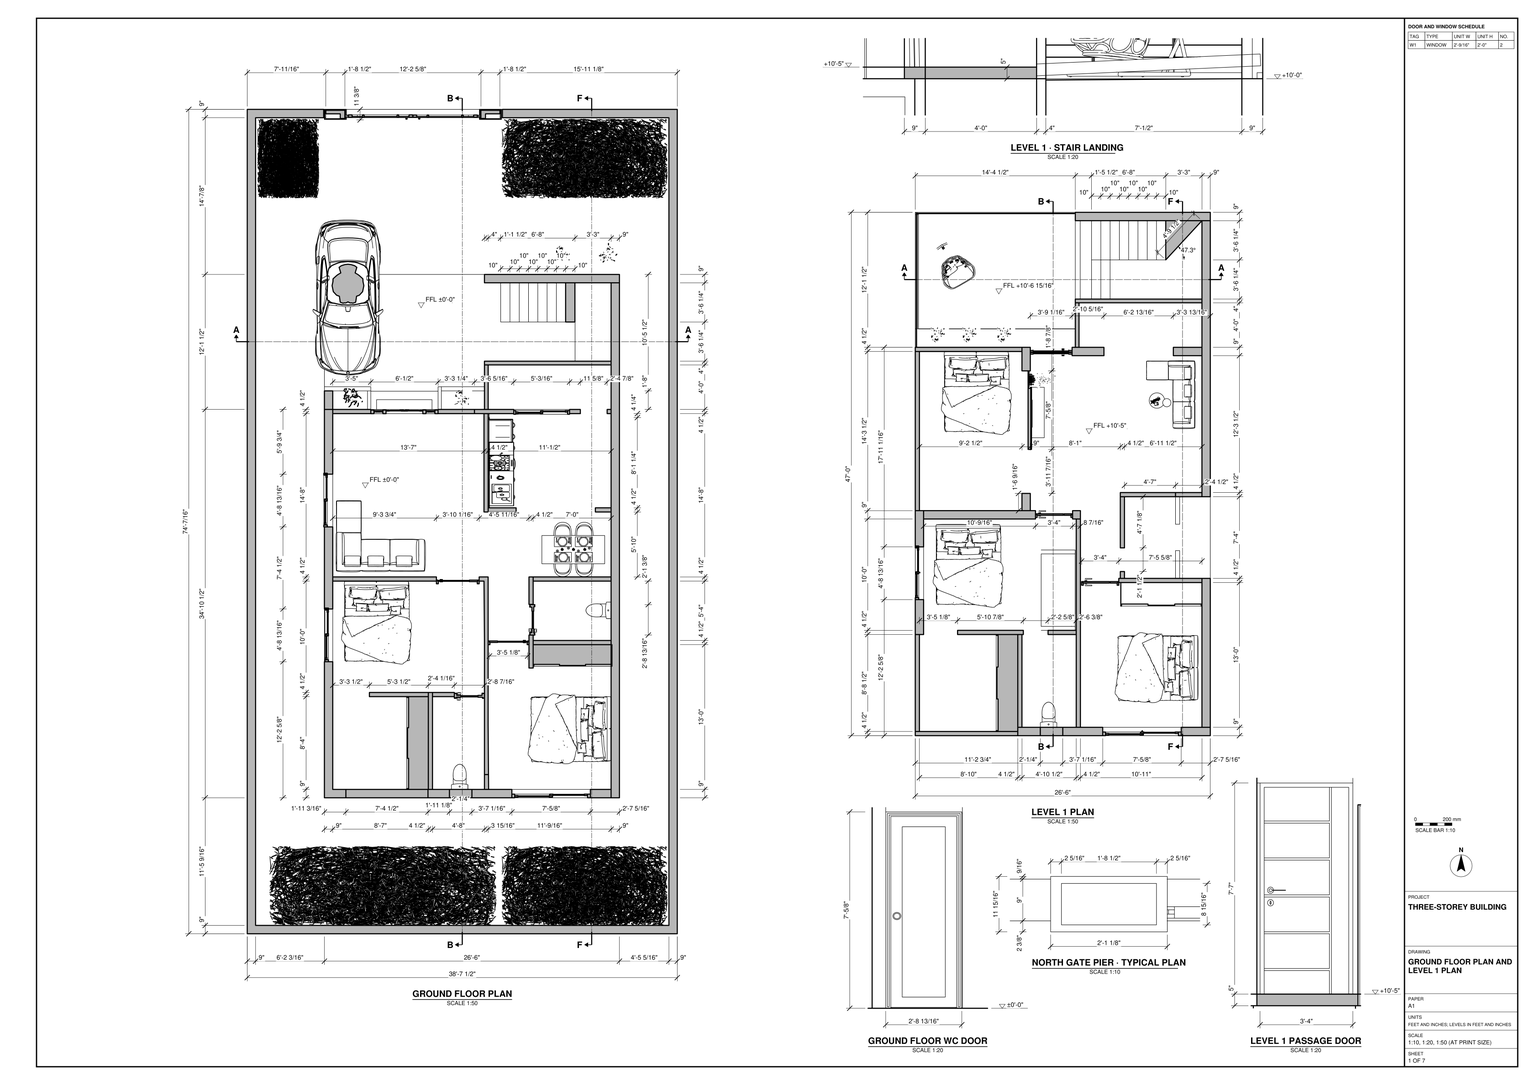
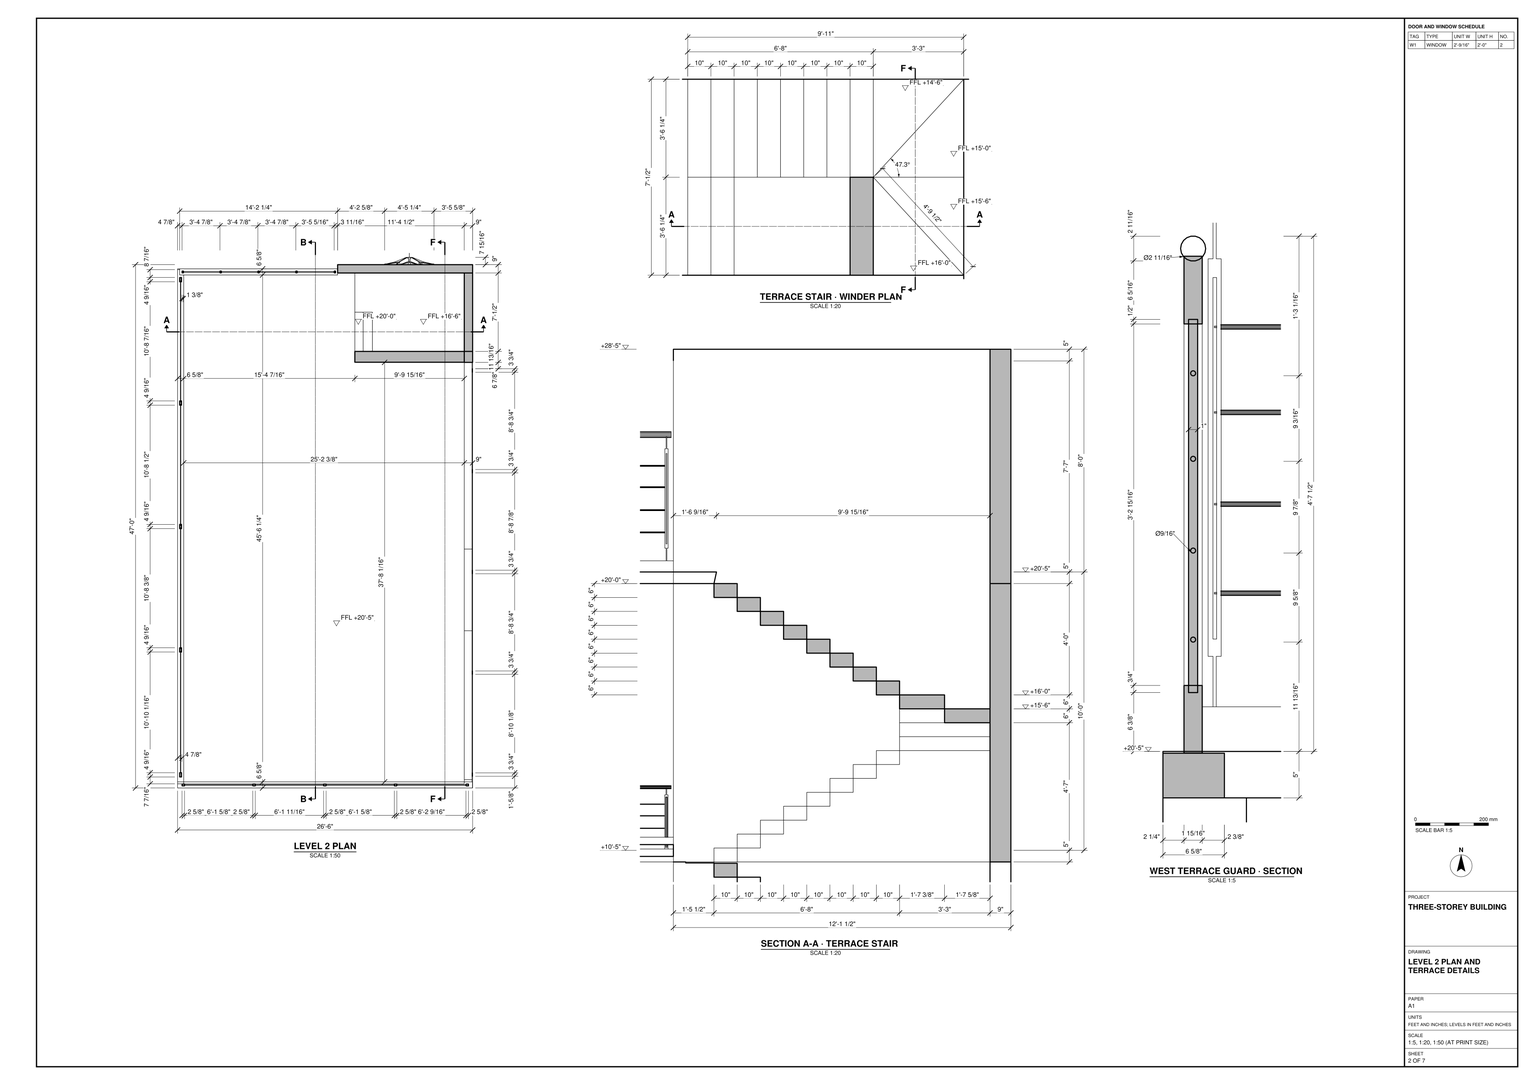
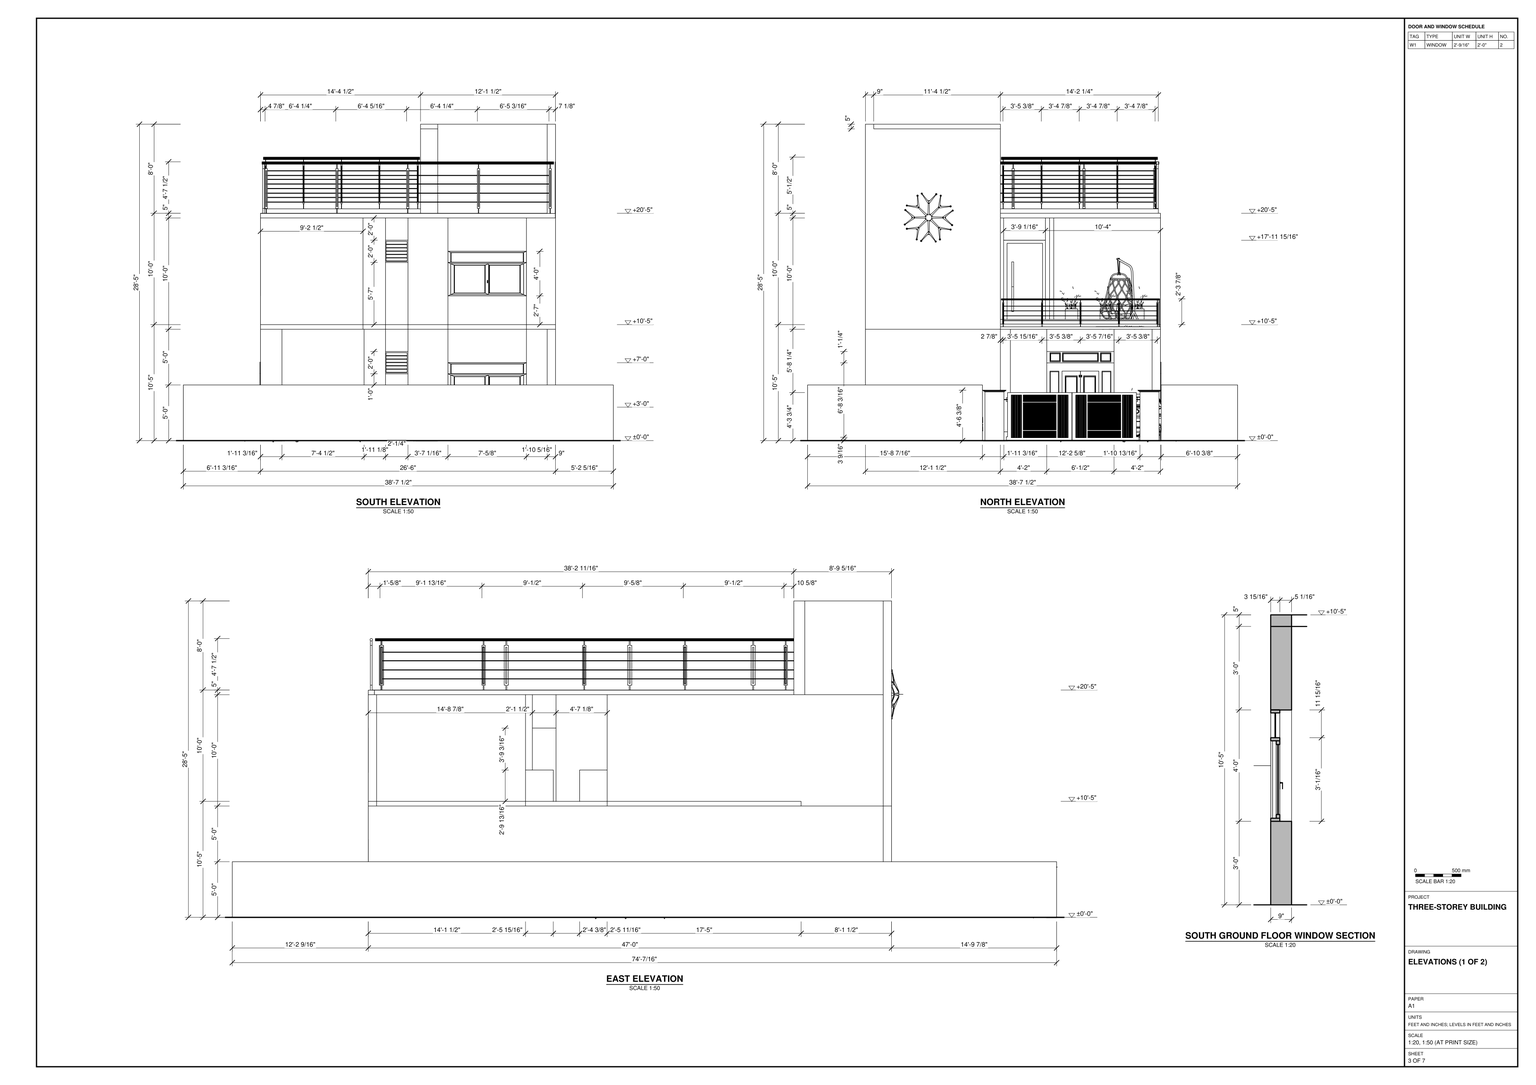
Use task_files/diagram_01.pdf to build the residence and its walled plot in SketchUp. Work in feet and inches. The model, including the site, measures 38'-7 1/2" across by 74'-1" from north to south, with an overall height of 28'-6 1/2". Set the ground floor at ±0'-0", Level 1 at +10'-5", and the Level 2 roof terrace at +20'-5".

Place the north entrance gate and its piers in line with the parking area. Leave the side passages and the planted areas at the north and south ends as drawn. Build the exterior walls and interior partitions to their respective plan thicknesses. Follow the plans for the lower-floor living, cooking, dining, sleeping and WC spaces, and for the bedrooms, sitting area and balcony on Level 1. Fit the doors and window units to the openings shown in plan and elevation. Include the kitchen counter, storage joinery, beds, sofas and dining furniture at their drawn sizes and positions.

Use the stair plans and sections to connect the landings, form the winder turn and carry the stair up through the terrace slab. Model the raised stair walls and the guards along the exposed terrace edges. Decor and loose items may be any suitable library components. Keep shell elements such as walls, slabs and roof, and each furniture or joinery piece, in separate groups or components; use components for repeated parts. Save one SketchUp model as output_files/three_storey_residence_with_a_roof_terrace.skp.

# SketchUp Ruby script. Lengths in inches.
U = 1.inch
M = Sketchup.active_model
def pt(a) = Geom::Point3d.new(a.map { |v| v * U })
def face(e, loops, mat)
  f = e.add_face(loops[0].map { |a| pt(a) })
  loops[1..].each { |l| e.add_face(l.map { |a| pt(a) }).erase! }
  f.material = f.back_material = mat if mat
  f
end
# faces: each face lists its corners as indices into pts; further lists are holes
def faces(e, pts, list, mat = nil) = list.each { |f| face(e, (f[0].is_a?(Array) ? f : [f]).map { |l| l.map { |i| pts[i] } }, mat) }
# xy, xz, yz: faces in a plane at the given z, y or x. An outline is a flat list of corners, or four numbers for a rectangle; further outlines are holes
def ring(l) = l.size == 4 ? [[l[0], l[1]], [l[2], l[1]], [l[2], l[3]], [l[0], l[3]]] : l.each_slice(2).to_a
def flat(e, list, mat, &to3) = list.each { |f| face(e, (f[0].is_a?(Array) ? f : [f]).map { |l| ring(l).map { |u, v| to3.(u, v) } }, mat) }
def xy(e, z, list, mat = nil) = flat(e, list, mat) { |x, y| [x, y, z] }
def xz(e, y, list, mat = nil) = flat(e, list, mat) { |x, z| [x, y, z] }
def yz(e, x, list, mat = nil) = flat(e, list, mat) { |y, z| [x, y, z] }
def lines(e, pts, list) = list.each { |a, b| e.add_line(pt(pts[a]), pt(pts[b])) }
# prism: a flat outline (further loops are holes) pulled along v
def prism(e, loops, v, mat = nil)
  f = face(e, loops, mat); d = Geom::Vector3d.new(v.map { |x| x * U })
  f.pushpull(f.normal.samedirection?(d) ? d.length : -d.length)
end
def box(e, o, s, mat = nil) = prism(e, [[o, [o[0] + s[0], o[1], o[2]], [o[0] + s[0], o[1] + s[1], o[2]], [o[0], o[1] + s[1], o[2]]]], [0, 0, s[2]], mat)
def at(x, y, z, deg = 0) = Geom::Transformation.translation(pt([x, y, z])) * Geom::Transformation.rotation(ORIGIN, Z_AXIS, deg.degrees)
def axes(o, x, y, z) = Geom::Transformation.new([*x, 0, *y, 0, *z, 0, *pt(o).to_a, 1])
def part(name) = M.definitions.add(name)
# library, detail: a bought-in or finely detailed component or shape, given as its bounding box
def library(name, o, s) = part(name).tap { |d| box(d.entities, o, s) }
def detail(e, o, s) = box(e.add_group.entities, o, s)
def put(e, d, t, mat = nil) = e.add_instance(d, t).tap { |i| i.material = mat if mat }
def group(e, t, mat = nil) = e.add_group.tap { |g| g.transformation = t; g.material = mat if mat }.entities
root = M.entities
M.materials.add("A02_Rose_Quartz").color = [255, 153, 153]
M.materials.add("B01_Ivory_Dust").color = [255, 217, 206]
M.materials.add("B02_Almond_Blush").color = [255, 177, 153]
M.materials.add("B05_Tangerine_Flame").color = [255, 59, 0]
M.materials.add("B07_Copper_Blaze").color = [153, 35, 0]
M.materials.add("C02_Golden_Beige").color = [255, 205, 155]
M.materials.add("C03_Honey_Glow").color = [255, 178, 101]
M.materials.add("C06_Saffron_Kiss").color = [204, 102, 0]
M.materials.add("C07_Caramel_Shine").color = [153, 76, 0]
M.materials.add("D01_Frost_White").color = [255, 242, 206]
M.materials.add("D04_Dandelion_Burst").color = [255, 204, 50]
M.materials.add("D05_Goldenrod_Hue").color = [255, 191, 0]
M.materials.add("D06_Sunflower_Bright").color = [204, 153, 0]
M.materials.add("E01_Mint_Frost").color = [255, 255, 204]
M.materials.add("Grass 2").color = [50, 81, 36]
M.materials.add("JJJ1").color = [238, 218, 183]
M.materials.add("MU TIGHI 6T67L 1").color = [235, 235, 235]
M.materials.add("T ER5Y 565N 1").color = [201, 111, 22]
M.materials.add("T R72 56 8, 7 5U1").color = [25, 25, 25]
M.materials.add("[Translucent_Glass_Gray]").color = [128, 128, 128]
M.materials["[Translucent_Glass_Gray]"].alpha = 0.5
M.materials.add("pyokki").color = [173, 96, 47]
M.materials.add("wefsd tger 1").color = [92, 92, 92]
c1 = library("CS300DRT",[0,0,0],[27.18,17.85,30.31])
c2 = library("Dining+Table",[-16.02,0,-0.16],[68,78.74,98.59])
c3 = library("michel-club1",[-34.67,-0.85,-0.13],[126.28,91.17,33.41])
c4 = library("Untitled+(2)",[-25.65,-58.99,0],[75.48,89.46,37.24])
c5 = library("Window with transom",[0,0,0],[5.2,55.12,70.87])
c6 = part("Group\#171")
p = [[0,43.31,5.11],[2.95,43.31,0],[2.95,0,0],[0,0,5.11]]
faces(c6.entities,p,[[0,1,2,3]],"[Translucent_Glass_Gray]")
c7 = part("Vwntilation+window (1)")
put(c7.entities,c6,at(43.48,1.97,32.29))
put(c7.entities,c6,at(43.48,1.97,26.38))
put(c7.entities,c6,at(43.48,1.97,20.48))
put(c7.entities,c6,at(43.48,1.97,14.57))
put(c7.entities,c6,at(43.48,1.97,8.67))
put(c7.entities,c6,at(43.48,1.97,2.76))
g1 = group(c7.entities,at(43.48,0,0))
prism(g1,[[[1.97,47.24,39.37],[1.97,0,39.37],[1.97,0,0],[1.97,47.24,0]],[[1.97,45.28,1.97],[1.97,1.97,1.97],[1.97,1.97,37.4],[1.97,45.28,37.4]]],[-1.97,0,0])
c8 = library("PINTU+6+YA",[0,-0.6875,0],[35.83,8.07,80.71])
c9 = library("T4592TW1\#2",[64.87,43.1,3.9375],[29.53,8.27,84.64])
c10 = library("car",[-8.95,-10.83,0],[83.51,184.88,55.74])
c11 = library("weed14.wee",[-333.89,-897.43,6.91],[387.4,250.53,60.12])
c12 = part("Grass")
put(c12.entities,c11,at(-109.53,-907.99,0),"Grass 2")
c13 = part("Box01")
box(c13.entities,[-251.12,-5.93,-8.91],[582.61,12.27,8.91],"wefsd tger 1")
c14 = part("Box45")
box(c14.entities,[-240.91,-0.82,12.1],[2.44,1.82,74.48],"JJJ1")
c15 = part("Cylinder01")
prism(c15.entities,[[[328.21,-1.16,98.56],[328.21,-0.34,98.26],[328.21,0.53,98.26],[328.21,1.34,98.56],[328.21,2.01,99.11],[328.21,2.44,99.87],[328.21,2.59,100.72],[328.21,2.44,101.58],[328.21,2.01,102.33],[328.21,1.34,102.89],[328.21,0.53,103.18],[328.21,-0.34,103.18],[328.21,-1.16,102.89],[328.21,-1.82,102.33],[328.21,-2.25,101.58],[328.21,-2.41,100.72],[328.21,-2.25,99.87],[328.21,-1.82,99.11]]],[-576.3,0,0],"T ER5Y 565N 1")
c16 = part("Cylinder02")
prism(c16.entities,[[[-239.93,0.18,76.32],[-239.93,0.34,76.26],[-239.93,0.48,76.15],[-239.93,0.5625,75.99],[-239.93,0.59,75.82],[-239.93,0.5625,75.65],[-239.93,0.48,75.5],[-239.93,0.34,75.39],[-239.93,0.18,75.33],[-239.93,0.01,75.33],[-239.93,-0.16,75.39],[-239.93,-0.29,75.5],[-239.93,-0.375,75.65],[-239.93,-0.41,75.82],[-239.93,-0.375,75.99],[-239.93,-0.29,76.15],[-239.93,-0.16,76.26],[-239.93,0.01,76.32]]],[560.05,0,0],"T R72 56 8, 7 5U1")
c17 = part("Rectangle1")
prism(c17.entities,[[[-237.41,1.91,10.08],[-239.22,1.91,10.08],[-239.22,1.91,0.02],[-240.41,1.91,0.02],[-240.41,1.91,10.08],[-242.22,1.91,10.08],[-242.22,1.91,89.41],[-240.41,1.91,89.41],[-240.41,1.91,99.1875],[-239.22,1.91,99.1875],[-239.22,1.91,89.41],[-237.41,1.91,89.41]],[[-240.4375,1.91,85.68],[-240.4375,1.91,13.53],[-239.08,1.91,13.53],[-239.08,1.91,85.68]]],[0,-3.64,0],"MU TIGHI 6T67L 1")
c18 = part("skp243")
put(c18.entities,c13,at(0,0,0))
put(c18.entities,c14,at(0,0,0))
put(c18.entities,c15,at(0,0,0))
put(c18.entities,c16,at(0,0,0))
put(c18.entities,c17,at(0,0,0))
put(c18.entities,c16,at(0,0,-17.07))
put(c18.entities,c16,at(0,0,-35.38))
put(c18.entities,c16,at(0,0,-53.15))
put(c18.entities,c14,at(139.83,0,0))
put(c18.entities,c17,at(139.83,0,0))
put(c18.entities,c17,at(279.78,0,0))
put(c18.entities,c14,at(279.78,0,0))
put(c18.entities,c14,at(419.57,0,0))
put(c18.entities,c17,at(419.57,0,0))
put(c18.entities,c17,at(561.11,0,0))
put(c18.entities,c14,at(561.11,0,0))
c19 = part("Railing1\#1")
put(c19.entities,c18,at(251.12,5.93,8.91))
c20 = part("Group\#41")
box(c20.entities,[0,0,0],[10,42.25,6])
c21 = part("Group\#46")
box(c21.entities,[0,0,0],[10,42.25,6])
c22 = library("Group\#56",[0,-0.9375,0],[208.49,31.89,113.57])
c23 = library("Group\#71",[0,0,0],[26.45,25.63,46.04])
c24 = library("Group\#72",[0,0,0],[26.45,25.63,49.07])
c25 = library("Group\#238",[0,0.18,0],[126.77,13.39,109.66])
c26 = part("Group\#245")
xy(c26.entities,0,[[0,0,0,23.23,0.63,23.23,0.63,23.11,71.02,23.11,71.02,23.23,71.65,23.23,71.65,0]])
xy(c26.entities,5.28,[[0.63,23.11,71.02,23.23]])
xy(c26.entities,5.91,[[0.63,21.26,24.02,21.26,24.02,22.44,47.64,22.44,47.64,21.26,71.02,21.26,71.02,23.23,0.63,23.23]])
xy(c26.entities,85.98,[[0.63,21.26,0.63,23.23,71.02,23.23,71.02,21.26,47.64,21.26,47.64,22.44,24.02,22.44,24.02,21.26]])
xy(c26.entities,86.61,[[0,0,0.63,23.23],[0.63,0,71.02,23.23],[71.02,0,71.65,23.23]])
xz(c26.entities,0,[[0,0,0.63,86.61],[0.63,0,71.02,85.98],[71.02,0,71.65,86.61],[0.63,85.98,71.02,86.61]])
xz(c26.entities,21.26,[[0.63,5.91,24.02,85.98],[47.64,5.91,71.02,85.98]])
xz(c26.entities,22.44,[[24.02,5.91,47.64,85.98]])
xz(c26.entities,23.11,[[0.63,0,71.02,5.28]])
xz(c26.entities,23.23,[[0,0,0.63,86.61],[71.02,0,71.65,86.61],[0.63,5.28,71.02,5.91],[0.63,85.98,71.02,86.61]])
yz(c26.entities,0,[[0,0,23.23,86.61]])
yz(c26.entities,0.63,[[23.11,0,23.23,5.28],[21.26,5.91,23.23,85.98]])
yz(c26.entities,24.02,[[21.26,5.91,22.44,85.98]])
yz(c26.entities,47.64,[[21.26,5.91,22.44,85.98]])
yz(c26.entities,71.02,[[23.11,0,23.23,5.28],[21.26,5.91,23.23,85.98]])
yz(c26.entities,71.65,[[0,0,23.23,86.61]])
c27 = library("Group\#280",[0,0,0],[192.97,36.5,79.04])
c28 = library("Group\#282",[0,0,0],[26.45,25.63,49.07])
c29 = library("Group\#281",[0,0,0],[26.45,25.63,46.04])
c30 = library("porta+de+madeira",[3.7,-4.82,1.36],[53.55,7.65,83.26])
c31 = library("Group\#287",[-2.43,-2.43,0],[21.3,21.3,3.83])
c32 = library("tv+unit",[8.62,4.37,0],[143.47,31.32,94.49])
c33 = library("C361",[153.37,-0.25,-0.8],[46.02,50.98,76.82])
c34 = library("Sofa",[-43.32,-37.8,0],[86.62,36.62,34.15])
c35 = part("Railing1")
put(c35.entities,c18,at(251.12,5.93,8.91))
c36 = part("Group\#159")
box(c36.entities,[0,0,0],[10,42.25,6])
c37 = part("Group\#164")
box(c37.entities,[0,0,0],[10,42.25,6])
c38 = library("Group\#240",[-1.79,0,0],[44.32,30.11,44.11])
c39 = library("Group\#283",[0,0,0],[26.45,25.63,46.14])
prism(root,[[[86.68,709.66,125.58],[86.68,585.05,120],[86.68,584.82,125.09],[86.68,709.4375,130.67]]],[168.98,0,0])
xy(root,0,[[[83.16,146.55,401.16,710.55],[255.66,171.58,259.625,171.61,259.625,171.58],[256.91,155.52,256.91,155.55,260.16,155.55]],[256.91,155.52,260.16,155.55,256.91,155.55],[255.66,171.58,259.625,171.58,259.625,171.61]])
xy(root,120,[[255.66,617.05,260.97,701.55]])
xy(root,240,[[83.16,151.05,83.16,706.05,273.16,706.05,273.16,617.05,392.16,617.05,392.16,151.05],[392.16,617.05,401.16,701.55]])
xy(root,245,[[83.16,151.05,392.16,151.05,392.16,605.375,274.23,605.375,274.23,706.05,83.16,706.05]])
xy(root,341,[[392.16,605.24,401.16,617.05],[255.66,605.375,274.23,605.375,274.23,617.05,392.16,617.05,392.16,710.55,255.66,710.55],[274.23,605.375,392.16,617.05],[392.16,617.05,401.16,701.55]])
xz(root,151.05,[[83.16,240,392.16,245]])
xz(root,605.24,[[392.16,240,401.16,341]])
xz(root,605.375,[[274.23,245,392.16,341],[255.66,336,274.23,341]])
xz(root,617.05,[[273.16,240,274.23,245,274.23,341,392.16,341,392.16,240],[392.16,240,401.16,341]])
xz(root,701.55,[[392.16,240,401.16,341]])
xz(root,706.05,[[83.16,240,83.16,245,274.23,245,273.16,240]])
xz(root,710.55,[[255.66,336,392.16,341]])
yz(root,83.16,[[151.05,240,706.05,245]])
yz(root,255.66,[[605.375,336,710.55,341]])
yz(root,274.23,[[605.375,245,617.05,341]])
yz(root,392.16,[[151.05,240,605.24,245],[605.24,240,617.05,240,617.05,341,605.375,341,605.375,245,605.24,245],[617.05,240,701.55,341],[605.24,245,605.375,341],[701.55,336,710.55,341]])
yz(root,401.16,[[605.24,240,617.05,341],[617.05,240,701.55,341]])
# 8 loose lines left out
p = [[260.97,617.05,119.43],[273.16,617.05,119.43],[273.16,701.55,120],[260.97,701.55,120],[274.23,617.05,245],[273.16,617.05,240],
  [273.16,706.05,240],[274.23,706.05,245]]
faces(root,p,[[0,1,2,3],[4,5,6,7]])
put(root,c1,axes([392.18,339.59,0],[-1,0,0],[0,1,0],[0,0,1]))
put(root,c2,axes([385.27,398.73,13.9375],[0,0.86,0],[-0.86,0,0],[0,0,0.86]))
put(root,c3,axes([122.14,466.0625,-1.4],[0.76405,0,0],[0,-0.84334,0],[0,0,0.7208]))
put(root,c4,at(127.23,349.58,0))
put(root,c4,at(361.69,232.99,0,-90))
put(root,c5,axes([369.82,146.55,36],[0,1,0],[-1.53511,0,0],[0,0,0.6784]))
put(root,c5,axes([83.76,351,36],[0.95488,0,0],[0,-1.04912,0],[0,0,0.68518]))
put(root,c5,axes([82.51,496.3,36],[0.95488,0,0],[0,-1.04912,0],[0,0,0.68518]))
put(root,c7,axes([242.16,172.11,72],[0,-0.52,0],[-0.52,0,0],[0,0,0.6096]))
put(root,c5,axes([347.41,559.85,36],[0,1,0],[-1.09194,0,0],[0,0,0.6784]))
put(root,c8,axes([303.66,311.6,0],[-1.22901,0,0],[0,1,0],[0,0,1.18946]))
put(root,c8,axes([203.88,377.17,0],[1.28577,0,0],[0,1,0],[0,0,1.18946]))
put(root,c9,axes([326.97,208.68,-3.9375],[-1.09935,0,0],[0,1,0],[0,0,1]))
put(root,c9,axes([355.03,426.73,-3.9375],[0,-1.11034,0],[-1,0,0],[0,0,1]))
put(root,c1,axes([220.05,155.55,0],[0,1,0],[1,0,0],[0,0,1]))
put(root,c10,axes([78.85,611.75,0],[0.90541,0,0],[0,0.90541,0],[0,0,0.90541]))
put(root,c12,axes([478.55,1406.72,4.77],[0.46,0,0],[0,0.34,0],[0,0,0.31]))
put(root,c12,axes([86.73,1406.72,4.77],[0.1702,0,0],[0,0.34,0],[0,0,0.31]))
put(root,c12,axes([478.55,622.84,4.77],[0.46,0,0],[0,0.34,0],[0,0,0.31]))
put(root,c12,axes([303.64,622.84,4.77],[0.6302,0,0],[0,0.34,0],[0,0,0.31]))
put(root,c19,axes([83.16,146.55,240],[0.5454,0,0],[0,0.54,0],[0,0,0.54]))
put(root,c19,axes([83.16,705.16,240],[0,-0.95109,0],[0.54,0,0],[0,0,0.54]))
put(root,c19,axes([401.16,605.24,240],[0,-0.77603,0],[-0.05181,0,0],[0,0,0.54]))
put(root,c19,axes([85.43,699.42,245],[0.29219,0,0],[0,0.54,0],[0,0,0.54]))
g2 = group(root,at(255.66,701.55,0))
xy(g2,0,[[0,0,145.5,9]])
xy(g2,120,[[0,0,145.5,9]])
xz(g2,0,[[0,0,136.5,120],[136.5,0,145.5,120]])
xz(g2,9,[[0,0,145.5,120]],"C02_Golden_Beige")
yz(g2,0,[[0,0,9,120]])
yz(g2,145.5,[[0,0,9,120]])
g3 = group(root,at(392.16,146.55,0))
xy(g3,0,[[0,0,9,555]])
xy(g3,120,[[0,0,9,555]])
xz(g3,0,[[0,0,9,120]])
xz(g3,555,[[0,0,9,120]])
yz(g3,0,[[0,0,9,120],[165,0,169.5,120],[169.5,0,233.5,120],[233.5,0,238,120],[307.99,0,312.49,120],
  [414,0,418.5,120],[418.5,0,466.5,120],[466.5,0,470.5,120],[470.5,0,555,120]])
yz(g3,0,[[9,0,165,120]],"A02_Rose_Quartz")
yz(g3,0,[[238,0,307.99,120]],"C07_Caramel_Shine")
yz(g3,0,[[312.49,0,414,120]],"D05_Goldenrod_Hue")
yz(g3,9,[[0,0,555,120]])
g4 = group(root,at(369.82,146.55,0))
xy(g4,0,[[0,0,22.34,9]])
xy(g4,120,[[0,0,22.34,9]])
xz(g4,0,[[0,0,22.34,120]])
xz(g4,9,[[0,0,22.34,120]],"A02_Rose_Quartz")
yz(g4,0,[[0,0,9,120]])
yz(g4,22.34,[[0,0,9,120]])
g5 = group(root,at(285.21,146.55,0))
xy(g5,0,[[0,0,84.61,9]])
xy(g5,36,[[0,0,84.61,9]])
xy(g5,84,[[0,0,84.61,9]])
xy(g5,120,[[0,0,84.61,9]])
xz(g5,0,[[0,0,84.61,36],[0,84,84.61,120]])
xz(g5,9,[[0,0,84.61,36],[0,84,84.61,120]],"A02_Rose_Quartz")
yz(g5,0,[[0,0,9,36],[0,84,9,120]])
yz(g5,84.61,[[0,0,9,36],[0,84,9,120]])
# 2 loose lines left out
g6 = group(root,at(242.16,146.55,0))
xy(g6,0,[[0,0,0,9,14.75,9,14.75,8.97,18,9,43.05,9,43.05,0]])
xy(g6,120,[[0,0,43.05,0,43.05,9,18,9,14.75,8.97,14.75,9,0,9]])
xz(g6,0,[[0,0,43.05,120]])
xz(g6,9,[[0,0,13.5,120],[13.5,0,14.75,120]])
xz(g6,9,[[18,0,43.05,120]],"A02_Rose_Quartz")
yz(g6,0,[[0,0,9,120]])
yz(g6,14.75,[[8.97,0,9,120]])
yz(g6,43.05,[[0,0,9,120]])
p = [[18,9,0],[14.75,8.97,0],[14.75,8.97,120],[18,9,120]]
faces(g6,p,[[0,1,2,3]])
g7 = group(root,at(217.92,146.55,0))
box(g7,[0,0,0],[24.24,9,72])
box(g7,[0,0,96],[24.24,9,24])
# 2 loose lines left out
g8 = group(root,at(194.8,146.55,0))
prism(g8,[[[23.13,0,0],[0,0,0],[0,9,0],[0.36,9,0],[4.86,9,0],[23.13,9,0]]],[0,0,120])
g9 = group(root,at(106.32,146.55,0))
xy(g9,0,[[0,0,88.48,9]])
xy(g9,120,[[0,0,88.48,9]])
xz(g9,0,[[0,0,88.48,120]])
xz(g9,9,[[0,0,88.48,120]],"B01_Ivory_Dust")
yz(g9,0,[[0,0,9,120]])
yz(g9,88.48,[[0,0,9,120]])
g10 = group(root,at(83.16,146.55,0))
xy(g10,0,[[0,0,0,146.63,9,146.63,9,9,23.16,9,23.16,0]])
xy(g10,120,[[0,0,23.16,0,23.16,9,9,9,9,146.63,0,146.63]])
xz(g10,0,[[0,0,23.16,120]])
xz(g10,9,[[9,0,23.16,120]],"B01_Ivory_Dust")
xz(g10,146.63,[[0,0,9,120]])
yz(g10,0,[[0,0,146.63,120]])
yz(g10,9,[[9,0,146.63,120]],"B01_Ivory_Dust")
yz(g10,23.16,[[0,0,9,120]])
g11 = group(root,at(83.16,293.18,0))
xy(g11,0,[[0,0,9,56.83]])
xy(g11,36,[[0,0,9,56.83]])
xy(g11,84,[[0,0,9,56.83]])
xy(g11,120,[[0,0,9,56.83]])
xz(g11,0,[[0,0,9,36],[0,84,9,120]])
xz(g11,56.83,[[0,0,9,36],[0,84,9,120]])
yz(g11,0,[[0,0,56.83,36],[0,84,56.83,120]])
yz(g11,9,[[0,0,56.83,36],[0,84,56.83,120]],"B01_Ivory_Dust")
# 2 loose lines left out
g12 = group(root,at(83.16,350,0))
xy(g12,0,[[0,0,9,88.47]])
xy(g12,120,[[0,0,9,88.47]])
xz(g12,0,[[0,0,9,120]])
xz(g12,88.47,[[0,0,9,120]])
yz(g12,0,[[0,0,88.47,120]])
yz(g12,9,[[30.05,0,34.55,120]])
yz(g12,9,[[0,0,30.05,120]],"B01_Ivory_Dust")
yz(g12,9,[[34.55,0,88.47,120]],"C02_Golden_Beige")
g13 = group(root,at(83.16,438.48,0))
xy(g13,0,[[0,0,9,56.83]])
xy(g13,36,[[0,0,9,56.83]])
xy(g13,84,[[0,0,9,56.83]])
xy(g13,120,[[0,0,9,56.83]])
xz(g13,0,[[0,0,9,36],[0,84,9,120]])
xz(g13,56.83,[[0,0,9,36],[0,84,9,120]])
yz(g13,0,[[0,0,56.83,36],[0,84,56.83,120]])
yz(g13,9,[[0,0,56.83,36],[0,84,56.83,120]],"C02_Golden_Beige")
# 2 loose lines left out
g14 = group(root,at(83.16,495.3,0))
xy(g14,0,[[0,0,9,69.75]])
xy(g14,120,[[0,0,9,69.75]])
xz(g14,0,[[0,0,9,120]])
xz(g14,69.75,[[0,0,9,120]])
yz(g14,0,[[0,0,69.75,120]])
yz(g14,9,[[0,0,69.75,120]],"C02_Golden_Beige")
g15 = group(root,at(83.16,565.05,0))
box(g15,[0,0,0],[9,20,120])
g16 = group(root,at(83.16,585.05,0))
prism(g16,[[[50,0,0],[46.46,0,0],[9,0,0],[0,0,0],[0,4.5,0],[50,4.5,0]]],[0,0,9.5])
g17 = group(root,at(129.62,565.05,0))
box(g17,[0,0,0],[3.54,20,9.5])
g18 = group(root,at(209.2,585.05,0))
box(g18,[0,0,0],[46.46,4.5,9.5])
g19 = group(root,at(205.66,565.05,0))
prism(g19,[[[0,24.5,0],[3.54,24.5,0],[3.54,20,0],[3.54,0,0],[0,0,0]]],[0,0,9.5])
g20 = group(root,at(167.55,560.55,0))
xy(g20,0,[[0,0,38.11,4.5]])
xy(g20,120,[[38.11,0,77.35,4.5]])
xz(g20,0,[[38.11,0,77.35,120]],"C02_Golden_Beige")
xz(g20,4.5,[[38.11,0,77.35,120]],"C02_Golden_Beige")
yz(g20,38.11,[[0,0,4.5,120]])
yz(g20,77.35,[[0,0,4.5,120]])
g21 = group(root,at(244.9,560.55,0))
prism(g21,[[[0,4.5,0],[10.76,4.5,0],[14.76,4.5,0],[42.33,4.5,0],[42.33,0,0],[14.76,0,0],[10.26,0,0],[0,0,0]]],[0,0,120],"C02_Golden_Beige")
g22 = group(root,at(255.16,454.54,0))
prism(g22,[[[4.5,4.5,0],[4.5,0,0],[0,0,0],[0,106.01,0],[4.5,106.01,0]]],[0,0,120],"C02_Golden_Beige")
g23 = group(root,at(259.66,454.54,0))
xy(g23,0,[[0,0,30.12,4.5]])
xy(g23,120,[[0,0,30.12,4.5]])
xz(g23,0,[[0,0,30.12,120]],"C02_Golden_Beige")
xz(g23,4.5,[[0,0,30.12,120]])
yz(g23,0,[[0,0,4.5,120]])
yz(g23,30.12,[[0,0,4.5,120]])
g24 = group(root,at(375.21,454.54,0))
xy(g24,0,[[0,0,16.95,4.5]])
xy(g24,120,[[0,0,16.95,4.5]])
xz(g24,0,[[0,0,16.95,120]],"C06_Saffron_Kiss")
xz(g24,4.5,[[0,0,16.95,120]])
yz(g24,0,[[0,0,4.5,120]])
yz(g24,16.95,[[0,0,4.5,120]])
g25 = group(root,at(308.16,380.05,0))
xy(g25,0,[[0,0,84,4.5]])
xy(g25,120,[[0,0,84,4.5]])
xz(g25,0,[[0,0,84,120]])
xz(g25,4.5,[[0,0,84,120]],"C07_Caramel_Shine")
yz(g25,0,[[0,0,4.5,120]])
yz(g25,84,[[0,0,4.5,120]])
g26 = group(root,at(303.66,361.91,0))
xy(g26,0,[[0,-6.96,4.5,22.64]])
xy(g26,120,[[0,-6.96,4.5,22.64]])
xz(g26,-6.96,[[0,0,4.5,120]])
xz(g26,22.64,[[0,0,4.5,120]])
yz(g26,0,[[-6.96,0,22.64,120]],"E01_Mint_Frost")
yz(g26,4.5,[[-6.96,0,18.14,120],[18.14,0,22.64,120]])
g27 = group(root,at(249.95,171.58,0))
xy(g27,0,[[5.71,0,5.71,144.47,5.31,196.04,5.21,208.47,0,208.47,0,212.97,9.67,212.97,9.67,52.45,10.08,0.03,9.67,0.03]])
xy(g27,120,[[5.71,0,9.67,0.03,10.08,0.03,9.67,52.45,9.67,212.97,0,212.97,0,208.47,5.21,208.47,5.31,196.04,5.71,144.47]])
xz(g27,0.03,[[9.67,0,10.08,120]])
xz(g27,208.47,[[0,0,5.21,120]])
xz(g27,212.97,[[0,0,9.67,120]],"C02_Golden_Beige")
yz(g27,0,[[208.47,0,212.97,120]])
yz(g27,5.71,[[0,0,144.47,120]],"B01_Ivory_Dust")
yz(g27,9.67,[[187.47,0,196.07,120],[196.07,0,212.97,120]])
yz(g27,9.67,[[52.45,0,187.47,120]],"A02_Rose_Quartz")
p = [[5.71,0,0],[9.67,0.03,0],[9.67,0.03,120],[5.71,0,120],[10.08,0.03,0],[9.67,52.45,0],
  [9.67,52.45,120],[10.08,0.03,120],[5.31,196.04,0],[5.71,144.47,0],[5.71,144.47,120],[5.31,196.04,120],
  [5.21,208.47,0],[5.21,208.47,120]]
faces(g27,p,[[0,1,2,3]])
faces(g27,p,[[4,5,6,7]],"A02_Rose_Quartz")
faces(g27,p,[[8,9,10,11],[12,8,11,13]],"B01_Ivory_Dust")
g28 = group(root,at(92.16,380.05,0))
xy(g28,0,[[0,0,111.72,4.5]])
xy(g28,120,[[0,0,111.72,4.5]])
xz(g28,0,[[0,0,111.72,120]],"B01_Ivory_Dust")
xz(g28,4.5,[[0,0,111.72,120]],"C02_Golden_Beige")
yz(g28,0,[[0,0,4.5,120]])
yz(g28,111.72,[[0,0,4.5,120]])
g29 = group(root,at(131.65,255.55,0))
box(g29,[0,0,0],[63.51,4.5,120],"D01_Frost_White")
g30 = group(root,at(199.66,155.55,0))
p = [[0,104.5,0],[0,0,0]]
lines(g30,p,[[0,1]])
g31 = group(root,at(255.66,155.55,0))
xy(g31,0,[[0,0,0,16.03,3.96,16.03,3.96,16.0625,4.375,16.0625,4.5,0]])
xy(g31,120,[[0,0,4.5,0,4.375,16.0625,3.96,16.0625,3.96,16.03,0,16.03]])
xz(g31,0,[[0,0,1.25,120],[1.25,0,4.5,120]])
xz(g31,16.03,[[0,0,3.96,120]])
xz(g31,16.0625,[[3.96,0,4.375,120]])
yz(g31,0,[[0,0,16.03,120]],"B01_Ivory_Dust")
yz(g31,3.96,[[16.03,0,16.0625,120]])
p = [[4.5,0,0],[4.375,16.0625,0],[4.375,16.0625,120],[4.5,0,120]]
faces(g31,p,[[0,1,2,3]],"A02_Rose_Quartz")
g32 = group(root,at(387.89,560.55,0))
box(g32,[0,0,0],[4.27,4.5,120])
g33 = group(root,at(347.41,560.55,0))
box(g33,[0,0,0],[11.61,4.5,120],"D05_Goldenrod_Hue")
g34 = group(root,at(287.23,560.55,0))
box(g34,[0,0,0],[60.19,4.5,36],"C02_Golden_Beige")
box(g34,[0,0,84],[60.19,4.5,36],"C02_Golden_Beige")
# 2 loose lines left out
g35 = group(root,at(255.66,565.05,0))
prism(g35,[[[0,24.5,0],[0,48,0],[4,48,0],[4,0,0],[0,0,0],[0,20,0]]],[0,0,120])
g36 = group(root,at(255.66,613.05,0))
prism(g36,[[[0,4,0],[136.5,4,0],[136.5,0,0],[4,0,0],[0,0,0]]],[0,0,120])
g37 = group(root,at(308.16,311.55,0))
xy(g37,0,[[0,0,84,4.5]])
xy(g37,120,[[0,0,84,4.5]])
xz(g37,0,[[0,0,84,120]],"A02_Rose_Quartz")
xz(g37,4.5,[[0,0,84,120]])
yz(g37,0,[[0,0,4.5,120]])
yz(g37,84,[[0,0,4.5,120]])
g38 = group(root,at(303.66,286.38,0))
prism(g38,[[[4.5,35.53,0],[4.5,29.67,0],[4.5,25.17,0],[4.5,0,0],[0,0,0],[0,35.53,0]]],[0,0,120],"E01_Mint_Frost")
g39 = group(root,at(195.16,155.55,0),"D01_Frost_White")
prism(g39,[[[0,0,0],[0,100,0],[0,104.5,0],[4.5,104.5,0],[4.5,0,0]]],[0,0,120],"D01_Frost_White")
g40 = group(root,at(139.39,565.05,0))
box(g40,[0,0,0],[59.74,10.56,7.05])
g41 = group(root,at(133.16,565.05,0))
prism(g41,[[[72.5,19.64,0],[72.5,0,0],[65.97,0,0],[65.97,10.56,0],[6.23,10.56,0],[6.23,0,0],[0,0,0],[0,19.64,0]]],[0,0,3.55])
put(root,c20,at(273.16,659.3,0))
put(root,c20,at(283.16,659.3,6))
put(root,c20,at(293.16,659.3,12))
put(root,c20,at(303.16,659.3,18))
put(root,c20,at(313.16,659.3,24))
put(root,c20,at(323.16,659.3,30))
put(root,c20,at(333.16,659.3,36))
put(root,c20,at(343.16,659.3,42))
g42 = group(root,at(353.16,659.3,48))
prism(g42,[[[39,42.25,0],[0,0,0],[0,42.25,0]]],[0,0,6])
g43 = group(root,at(353.16,659.3,54))
prism(g43,[[[39,0,0],[0,0,0],[39,42.25,0]]],[0,0,6])
g44 = group(root,at(353.16,617.05,60))
prism(g44,[[[39,0,0],[0,42.25,0],[39,42.25,0]]],[0,0,6])
g45 = group(root,at(353.16,617.05,65.43))
prism(g45,[[[0,42.25,0],[39,0,0],[0,0,0]]],[0,0,6])
put(root,c21,at(343.16,617.05,71.43))
put(root,c21,at(333.16,617.05,77.43))
put(root,c21,at(323.16,617.05,83.43))
put(root,c21,at(313.16,617.05,89.43))
put(root,c21,at(303.16,617.05,95.43))
put(root,c21,at(293.16,617.05,101.43))
put(root,c21,at(283.16,617.05,107.43))
put(root,c21,at(273.16,617.05,113.43))
put(root,c22,axes([291.97,459.04,0],[0,0.48687,0],[-1.044,0,0],[0,0,0.98784]))
put(root,c23,at(218,563.92,0))
put(root,c24,at(99.06,565.05,7.65))
g46 = group(root,at(260.16,311.55,0))
xy(g46,96,[[-0.54,0,43.5,4.5]])
xy(g46,120,[[-0.54,0,43.5,4.5]])
xz(g46,0,[[-0.54,96,43.5,120]],"A02_Rose_Quartz")
xz(g46,4.5,[[-0.54,96,43.5,120]])
yz(g46,-0.54,[[0,96,4.5,120]])
yz(g46,43.5,[[0,96,4.5,120]])
g47 = group(root,at(203.88,380.05,0))
xy(g47,96,[[0,0,46.07,4.5]])
xy(g47,120,[[0,0,46.07,4.5]])
xz(g47,0,[[0,96,46.07,120]],"B01_Ivory_Dust")
xz(g47,4.5,[[0,96,46.07,120]],"C02_Golden_Beige")
yz(g47,0,[[0,96,4.5,120]])
yz(g47,46.07,[[0,96,4.5,120]])
g48 = group(root,at(223.2,255.55,0))
box(g48,[0,0,84],[32.46,4.5,36],"D01_Frost_White")
g49 = group(root,at(199.66,255.55,0))
xy(g49,0,[[0,0,23.54,4.5]])
xy(g49,120,[[0,0,23.54,4.5]])
xz(g49,0,[[0,0,23.54,120]],"B01_Ivory_Dust")
xz(g49,4.5,[[0,0,23.54,120]],"D01_Frost_White")
yz(g49,0,[[0,0,4.5,120]])
yz(g49,23.54,[[0,0,4.5,120]])
g50 = group(root,at(303.66,321.91,0))
xy(g50,84,[[0,0,4.5,33.04]])
xy(g50,120,[[0,0,4.5,33.04]])
xz(g50,0,[[0,84,4.5,120]])
xz(g50,33.04,[[0,84,4.5,120]])
yz(g50,0,[[0,84,33.04,120]],"E01_Mint_Frost")
yz(g50,4.5,[[0,84,33.04,120]])
g51 = group(root,at(92.16,560.55,0))
xy(g51,0,[[0,0,41,4.5]])
xy(g51,120,[[0,0,41,4.5]])
xz(g51,0,[[0,0,41,120]],"C02_Golden_Beige")
xz(g51,4.5,[[0,0,41,120]],"C02_Golden_Beige")
yz(g51,0,[[0,0,4.5,120]])
yz(g51,41,[[0,0,4.5,120]])
g52 = group(root,at(133.16,560.55,0))
box(g52,[0,0,0],[72.5,4.5,3.55])
xy(g52,96,[[0,0,72.5,4.5]])
xy(g52,120,[[0,0,72.5,4.5]])
xz(g52,0,[[0,96,72.5,120]],"C02_Golden_Beige")
xz(g52,4.5,[[0,96,72.5,120]],"C02_Golden_Beige")
yz(g52,0,[[0,96,4.5,120]])
yz(g52,72.5,[[0,96,4.5,120]])
# 2 loose lines left out
put(root,c25,axes([133.16,564.94,3.55],[0.57189,0,0],[0,-0.329,0],[0,0,0.84304]))
put(root,c26,axes([195.16,155.55,0],[0,1.3956,0],[-1,0,0],[0,0,1]),"pyokki")
put(root,c26,axes([393.04,311.55,0],[-1.18458,0,0],[0,-1,0],[0,0,1]),"pyokki")
g53 = group(root,at(0,0,0))
xy(g53,0,[[[9,9,454.48,879.45],[83.16,146.55,401.16,710.55]],[82.375,879.45,275.03,888.45]])
xy(g53,60,[[0,0,463.48,0,463.48,888.45,275.03,888.45,275.03,879.45,454.48,879.45,454.48,9,9,9,9,879.45,82.375,879.45,82.375,888.45,0,888.45]])
xz(g53,0,[[0,0,463.48,60]])
xz(g53,9,[[9,0,454.48,60]])
xz(g53,879.45,[[9,0,82.375,60],[275.03,0,454.48,60]])
xz(g53,888.45,[[0,0,82.375,60],[275.03,0,463.48,60]])
yz(g53,0,[[0,0,888.45,60]])
yz(g53,9,[[9,0,879.45,60]])
yz(g53,82.375,[[879.45,0,888.45,60]])
yz(g53,275.03,[[879.45,0,888.45,60]])
yz(g53,454.48,[[9,0,879.45,60]])
yz(g53,463.48,[[0,0,888.45,60]])
put(root,c27,axes([66.29,863.47,-0.93],[1.0798,0,0],[0,0.7,0],[0,0,0.7]))
put(root,c28,at(374.49,718.88,0))
put(root,c29,at(326.51,719.32,0))
g54 = group(root,at(83.16,146.55,120))
prism(g54,[[[0,0,0],[0,438.5,0],[176.5,438.5,0],[176.5,466.5,0],[318,466.5,0],[318,0,0]]],[0,0,5])
g55 = group(root,at(627.52,146.55,118))
g56 = group(g55,at(-544.36,0,-1))
put(g56,c3,axes([249.53,383.97,3.08],[0,-0.58,0],[0.58,0,0],[0,0,0.58]))
put(g56,c4,at(274.35,85.37,3,-90))
put(g56,c5,axes([286.66,0,39],[0,1,0],[-1.53511,0,0],[0,0,0.6784]))
put(g56,c30,axes([120.89,415.17,1.43],[0.84104,0,0],[0,1.17577,0],[0,0,1.15304]))
put(g56,c7,axes([159,25.5625,75],[0,-0.52,0],[-0.52,0,0],[0,0,0.6096]))
put(g56,c8,axes([179.37,162.12,3],[1.11639,0,0],[0,1,0],[0,0,1.18946]))
put(g56,c1,at(152.61,9,3,90))
put(g56,c8,axes([129.59,235.12,3],[1.11639,0,0],[0,1,0],[0,0,1.18946]))
put(g56,c4,at(44.92,197.27,3))
put(g56,c5,axes([0,204.45,39],[0.95488,0,0],[0,-1.04912,0],[0,0,0.68518]))
put(g56,c31,axes([276.39,576.4,150.02],[-3.24,0,0],[0,0,-3.24],[0,-3.24,0]))
put(g56,c32,axes([117.24,398.22,3],[0,-0.59,0],[1,0,0],[0,0,1.03]))
put(g56,c33,at(-99.92,398.1,3.8,30))
put(g56,c4,at(53.77,383.53,3))
put(g56,c34,at(173.5,156.8,3,-90))
put(g56,c35,axes([2.45,418.5,3],[0,0.24871,0],[-0.2,0,0],[0,0,0.294]))
put(g56,c35,axes([0,561.55,3],[0.29608,0,0],[0,0.2,0],[0,0,0.2938]))
put(g56,c36,at(260,512.75,45))
g57 = group(g56,at(270,512.75,51))
prism(g57,[[[39,42.25,0],[0,0,0],[0,42.25,0]]],[0,0,6])
g58 = group(g56,at(110.5,0,3))
prism(g58,[[[24.26,0,0],[0,0,0],[0,4.5,0],[0,9,0],[4.5,9,0],[24.26,9,0]]],[0,0,120])
put(g56,c36,at(190,512.75,3))
put(g56,c36,at(210,512.75,15))
g59 = group(g56,at(270,512.75,57))
prism(g59,[[[39,0,0],[0,0,0],[39,42.25,0]]],[0,0,6])
g60 = group(g56,at(176.5,466.5,3))
p = [[0,0,0],[132.5,0,0]]
lines(g60,p,[[0,1]])
g61 = group(g56,at(4.5,242.5,3))
p = [[0,171.5,0],[0,0,0]]
lines(g61,p,[[0,1]])
g62 = group(g56,at(0,4.5,3))
xy(g62,0,[[0,0,4.5,104.5]])
xy(g62,120,[[0,0,4.5,104.5]])
xz(g62,0,[[0,0,4.5,120]])
xz(g62,104.5,[[0,0,4.5,120]])
yz(g62,0,[[0,0,104.5,120]])
yz(g62,4.5,[[0,0,104.5,120]],"B02_Almond_Blush")
g63 = group(g56,at(45.6,109,3))
xy(g63,0,[[0,0,70.89,4.5]])
xy(g63,120,[[0,0,70.89,4.5]])
xz(g63,0,[[64.9,0,69.4,120],[69.4,0,70.89,120]])
xz(g63,0,[[0,0,64.9,120]],"B02_Almond_Blush")
xz(g63,4.5,[[0,0,70.89,120]],"C03_Honey_Glow")
yz(g63,0,[[0,0,4.5,120]])
yz(g63,70.89,[[0,0,4.5,120]])
g64 = group(g56,at(0,146.63,3))
xy(g64,0,[[0,0,9,56.83]])
xy(g64,36,[[0,0,9,56.83]])
xy(g64,84,[[0,0,9,56.83]])
xy(g64,120,[[0,0,9,56.83]])
xz(g64,0,[[0,0,9,36],[0,84,9,120]])
xz(g64,56.83,[[0,0,9,36],[0,84,9,120]])
yz(g64,0,[[0,0,56.83,36],[0,84,56.83,120]])
yz(g64,9,[[0,0,56.83,36],[0,84,56.83,120]],"C03_Honey_Glow")
# 2 loose lines left out
g65 = group(g56,at(9,233.5,3))
xy(g65,0,[[0,0,120.59,9]])
xy(g65,120,[[0,0,120.59,9]])
xz(g65,0,[[0,0,120.59,120]],"C03_Honey_Glow")
xz(g65,9,[[106,0,115,120]])
xz(g65,9,[[0,0,106,120]],"B05_Tangerine_Flame")
xz(g65,9,[[115,0,120.59,120]],"D04_Dandelion_Burst")
yz(g65,0,[[0,0,9,120]])
yz(g65,120.59,[[0,0,9,120]],"D04_Dandelion_Burst")
g66 = group(g56,at(221,202.39,3))
box(g66,[0,0,0],[4.5,55.11,120])
g67 = group(g56,at(110.5,9,3))
xy(g67,0,[[0,0,4.5,100]])
xy(g67,120,[[0,0,4.5,100]])
xz(g67,0,[[0,0,4.5,120]])
xz(g67,100,[[0,0,4.5,120]])
yz(g67,0,[[0,0,100,120]],"B02_Almond_Blush")
yz(g67,4.5,[[0,0,100,120]])
g68 = group(g56,at(309,9,3))
xy(g68,0,[[0,0,9,160.5],[0,248.5,9,546]])
xy(g68,120,[[0,0,9,160.5],[0,248.5,9,546]])
xz(g68,0,[[0,0,9,120]])
xz(g68,160.5,[[0,0,9,120]])
xz(g68,248.5,[[0,0,9,120]])
xz(g68,546,[[0,0,9,120]])
yz(g68,0,[[156,0,160.5,120],[248.5,0,253,120],[400.5,0,409.5,120],[409.5,0,457.5,120],[457.5,0,461.5,120],
  [461.5,0,546,120]])
yz(g68,0,[[0,0,156,120]],"B07_Copper_Blaze")
yz(g68,0,[[253,0,400.5,120]],"D04_Dandelion_Burst")
yz(g68,9,[[0,0,160.5,120],[248.5,0,546,120]])
# 2 loose lines left out
g69 = group(g56,at(115,242.5,3))
xy(g69,0,[[0,0,9,18.56]])
xy(g69,120,[[0,0,9,18.56]])
xz(g69,0,[[0,0,9,120]])
xz(g69,18.56,[[0,0,9,120]])
yz(g69,0,[[0,0,18.56,120]],"B05_Tangerine_Flame")
yz(g69,9,[[0,0,18.56,120]],"D04_Dandelion_Burst")
g70 = group(g56,at(280.5,199.45,3))
xy(g70,0,[[0,0,4.5,28.38]])
g71 = group(g56,at(221,169.5,3))
box(g71,[0,0,0],[4.5,7.38,120])
g72 = group(g56,at(172.5,555,3))
xy(g72,0,[[0,0,145.5,9]])
xy(g72,221,[[0,0,145.5,9]])
xz(g72,0,[[0,0,136.5,221],[136.5,0,145.5,221]])
xz(g72,9,[[0,0,145.5,221]],"D06_Sunflower_Bright")
yz(g72,0,[[0,0,4.5,221],[4.5,0,9,221]])
yz(g72,145.5,[[0,0,9,221]])
g73 = group(g56,at(203.38,409.5,3))
xy(g73,0,[[0,0,74.8,9]])
g74 = group(g56,at(0,203.45,3))
xy(g74,0,[[0,0,9,39.05]])
xy(g74,120,[[0,0,9,39.05]])
xz(g74,0,[[0,0,9,120]])
xz(g74,39.05,[[0,0,4.5,120],[4.5,0,9,120]])
yz(g74,0,[[0,0,39.05,120]])
yz(g74,9,[[30.05,0,39.05,120]])
yz(g74,9,[[0,0,30.05,120]],"C03_Honey_Glow")
g75 = group(g56,at(278.18,409.5,3))
xy(g75,0,[[0,0,30.82,9]])
xy(g75,120,[[0,0,30.82,9]])
xz(g75,0,[[0,0,30.82,120]],"D04_Dandelion_Burst")
xz(g75,9,[[0,0,30.82,120]])
yz(g75,0,[[0,0,9,120]])
yz(g75,30.82,[[0,0,9,120]])
g76 = group(g56,at(115,393.14,3))
xy(g76,0,[[0,0,9,25.36]])
xy(g76,96.48,[[0,-132.08,9,0]])
xy(g76,120,[[0,-132.08,9,25.36]])
xz(g76,-132.08,[[0,96.48,9,120]])
xz(g76,0,[[0,0,9,96.48]])
xz(g76,25.36,[[0,0,4.5,120],[4.5,0,9,120]],"C07_Caramel_Shine")
yz(g76,0,[[20.86,0,25.36,120]])
yz(g76,0,[[0,0,0,96.48,-132.08,96.48,-132.08,120,20.86,120,20.86,0]],"B05_Tangerine_Flame")
yz(g76,9,[[0,0,25.36,0,25.36,120,-132.08,120,-132.08,96.48,0,96.48]],"D04_Dandelion_Burst")
# 1 loose lines left out
g77 = group(g56,at(221,257.5,3))
xy(g77,0,[[0,0,59.5,4.5]])
xy(g77,120,[[0,0,59.5,4.5]])
xz(g77,0,[[0,0,4.5,120],[4.5,0,59.5,120]])
xz(g77,4.5,[[0,0,59.5,120]],"D04_Dandelion_Burst")
yz(g77,0,[[0,0,4.5,120]])
yz(g77,59.5,[[0,0,4.5,120]])
g78 = group(g56,at(219.37,165,3))
xy(g78,0,[[0,0,89.63,4.5]])
xy(g78,120,[[0,0,89.63,4.5]])
xz(g78,0,[[0,0,89.63,120]],"B07_Copper_Blaze")
xz(g78,4.5,[[0,0,1.63,120],[1.63,0,6.13,120],[6.13,0,61.13,120],[61.13,0,65.63,120],[65.63,0,89.63,120]])
yz(g78,0,[[0,0,4.5,120]])
yz(g78,89.63,[[0,0,4.5,120]])
g79 = group(g56,at(286.66,0,3))
xy(g79,0,[[0,0,31.34,9]])
xy(g79,120,[[0,0,31.34,9]])
xz(g79,0,[[0,0,31.34,120]])
xz(g79,9,[[22.34,0,31.34,120]])
xz(g79,9,[[0,0,22.34,120]],"B07_Copper_Blaze")
yz(g79,0,[[0,0,9,120]])
yz(g79,31.34,[[0,0,9,120]])
g80 = group(g56,at(169.04,409.5,3))
prism(g80,[[[3.46,9,0],[7.46,9,0],[34.34,9,0],[34.34,0,0],[0,0,0],[0,9,0]]],[0,0,120],"D04_Dandelion_Burst")
g81 = group(g56,at(0,414,3))
xy(g81,0,[[0,0,115,4.5]])
xy(g81,120,[[0,0,115,4.5]])
xz(g81,0,[[0,0,4.5,120]])
xz(g81,0,[[4.5,0,115,120]],"B05_Tangerine_Flame")
xz(g81,4.5,[[0,0,115,120]],"C07_Caramel_Shine")
yz(g81,0,[[0,0,4.5,120]])
yz(g81,115,[[0,0,4.5,120]])
g82 = group(g56,at(172.5,418.5,3))
box(g82,[0,0,0],[4,48,120])
g83 = group(g56,at(202.05,0,3))
xy(g83,0,[[0,0,84.61,9]])
xy(g83,36,[[0,0,84.61,9]])
xy(g83,84,[[0,0,84.61,9]])
xy(g83,120,[[0,0,84.61,9]])
xz(g83,0,[[0,0,84.61,36],[0,84,84.61,120]])
xz(g83,9,[[0,0,84.61,36],[0,84,84.61,120]],"B07_Copper_Blaze")
yz(g83,0,[[0,0,9,36],[0,84,9,120]])
yz(g83,84.61,[[0,0,9,36],[0,84,9,120]])
# 2 loose lines left out
put(g56,c36,at(220,512.75,21))
put(g56,c36,at(230,512.75,27))
put(g56,c36,at(240,512.75,33))
put(g56,c36,at(200,512.75,9))
g84 = group(g56,at(0,109,3))
xy(g84,0,[[0,0,9,37.63]])
xy(g84,120,[[0,0,9,37.63]])
xz(g84,0,[[0,0,4.5,120],[4.5,0,9,120]])
xz(g84,37.63,[[0,0,9,120]])
yz(g84,0,[[0,0,37.63,120]])
yz(g84,9,[[0,0,37.63,120]],"C03_Honey_Glow")
g85 = group(g56,at(173.5,9,3))
xy(g85,0,[[0,0,4.5,224.5]])
xy(g85,120,[[0,0,4.5,224.5]])
xz(g85,0,[[0,0,4.5,120]])
xz(g85,224.5,[[0,0,4.5,120]])
yz(g85,0,[[0,0,100,120],[100,0,104.5,120]])
yz(g85,0,[[104.5,0,224.5,120]],"C03_Honey_Glow")
yz(g85,4.5,[[0,0,224.5,120]],"B07_Copper_Blaze")
g86 = group(g56,at(280.5,257.5,3))
xy(g86,0,[[0,0,28.5,4.5]])
xy(g86,120,[[0,0,28.5,4.5]])
xz(g86,0,[[0,0,4.5,120],[4.5,0,28.5,120]])
xz(g86,4.5,[[0,0,28.5,120]],"D04_Dandelion_Burst")
yz(g86,0,[[0,0,4.5,120]])
yz(g86,28.5,[[0,0,4.5,120]])
g87 = group(g56,at(0,0,3))
xy(g87,0,[[0,0,110.5,4.5]])
xy(g87,120,[[0,0,110.5,4.5]])
xz(g87,0,[[0,0,110.5,120]])
xz(g87,4.5,[[0,0,4.5,120]])
xz(g87,4.5,[[4.5,0,110.5,120]],"B02_Almond_Blush")
yz(g87,0,[[0,0,4.5,120]])
yz(g87,110.5,[[0,0,4.5,120]])
g88 = group(g56,at(159,0,3))
xy(g88,0,[[0,0,43.05,9]])
xy(g88,120,[[0,0,43.05,9]])
xz(g88,0,[[0,0,43.05,120]])
xz(g88,9,[[0,0,14.5,120],[14.5,0,19,120]])
xz(g88,9,[[19,0,43.05,120]],"B07_Copper_Blaze")
yz(g88,0,[[0,0,9,120]])
yz(g88,43.05,[[0,0,9,120]])
g89 = group(g56,at(169.59,233.5,3))
xy(g89,0,[[0,0,8.41,9]])
xy(g89,120,[[0,0,8.41,9]])
xz(g89,0,[[0,0,3.91,120],[3.91,0,8.41,120]])
xz(g89,9,[[0,0,8.41,120]],"D04_Dandelion_Burst")
yz(g89,0,[[0,0,9,120]])
yz(g89,8.41,[[0,0,9,120]])
g90 = group(g56,at(143.14,109,3))
xy(g90,0,[[0,0,30.36,4.5]])
xy(g90,120,[[0,0,30.36,4.5]])
xz(g90,0,[[0,0,30.36,120]])
xz(g90,4.5,[[0,0,30.36,120]],"C03_Honey_Glow")
yz(g90,0,[[0,0,4.5,120]])
yz(g90,30.36,[[0,0,4.5,120]])
g91 = group(g56,at(280.5,169.5,3))
box(g91,[0,0,0],[4.5,29.95,38.8])
put(g56,c36,at(250,512.75,39))
g92 = group(g56,at(270,470.5,69))
prism(g92,[[[0,42.25,0],[39,0,0],[0,0,0]]],[0,0,6])
put(g56,c37,at(250,470.5,81))
put(g56,c37,at(240,470.5,87))
put(g56,c37,at(230,470.5,93))
put(g56,c37,at(220,470.5,99))
put(g56,c37,at(210,470.5,105))
g93 = group(g56,at(270,470.5,63))
prism(g93,[[[39,0,0],[0,42.25,0],[39,42.25,0]]],[0,0,6])
put(g56,c37,at(260,470.5,75))
g94 = group(g56,at(129.59,233.5,3))
xy(g94,96,[[0,0,40,9]])
xy(g94,120,[[0,0,40,9]])
xz(g94,0,[[0,96,40,120]],"C03_Honey_Glow")
xz(g94,9,[[0,96,40,120]],"D04_Dandelion_Burst")
yz(g94,0,[[0,96,9,120]])
yz(g94,40,[[0,96,9,120]])
g95 = group(g56,at(221,176.88,3))
box(g95,[0,0,84],[4.5,25.51,36])
g96 = group(g56,at(0,242.5,3))
xy(g96,0,[[0,0,4.5,171.5]])
xy(g96,120,[[0,0,4.5,171.5]])
xz(g96,0,[[0,0,4.5,120]])
xz(g96,171.5,[[0,0,4.5,120]])
yz(g96,0,[[0,0,171.5,120]])
yz(g96,4.5,[[0,0,171.5,120]],"B05_Tangerine_Flame")
put(g56,c37,at(200,470.5,111))
g97 = group(g56,at(134.76,0,3))
box(g97,[0,0,0],[24.24,9,72])
box(g97,[0,0,96],[24.24,9,24])
# 2 loose lines left out
g98 = group(g56,at(280.5,227.84,3))
box(g98,[0,0,0],[4.5,29.66,38.8])
g99 = group(g56,at(116.49,109,3))
xy(g99,84,[[0,0,26.65,4.5]])
xy(g99,120,[[0,0,26.65,4.5]])
xz(g99,0,[[0,84,26.65,120]])
xz(g99,4.5,[[0,84,26.65,120]],"C03_Honey_Glow")
yz(g99,0,[[0,84,4.5,120]])
yz(g99,26.65,[[0,84,4.5,120]])
g100 = group(g56,at(172.5,466.5,3))
prism(g100,[[[4,0,0],[0,0,0],[0,4,0],[57.5,4,0],[67.5,4,0],[97.5,4,0],[136.5,4,0],[136.5,0,0]]],[0,0,120])
g101 = group(g56,at(178,165,3))
xy(g101,96,[[0,0,41.37,4.5]])
xy(g101,120,[[0,0,41.37,4.5]])
xz(g101,0,[[0,96,41.37,120]],"B07_Copper_Blaze")
xz(g101,4.5,[[0,96,41.37,120]])
yz(g101,0,[[0,96,4.5,120]])
yz(g101,41.37,[[0,96,4.5,120]])
put(g56,c37,at(190,470.5,117))
g102 = group(g56,at(124,409.5,3))
xy(g102,96,[[0,0,45.04,9]])
xy(g102,120,[[0,0,45.04,9]])
xz(g102,0,[[0,96,45.04,120]],"D04_Dandelion_Burst")
xz(g102,9,[[0,96,45.04,120]],"C07_Caramel_Shine")
yz(g102,0,[[0,96,9,120]])
yz(g102,45.04,[[0,96,9,120]])
g103 = group(g56,at(110.5,4.5,3),"pyokki")
xy(g103,0,[[-23.23,0,-23.23,0.92,-23.11,0.92,-23.11,103.58,-23.23,103.58,-23.23,104.5,0,104.5,0,0]])
xy(g103,5.28,[[-23.23,0.92,-23.11,103.58]])
xy(g103,5.91,[[-23.23,0.92,-21.26,0.92,-21.26,35.02,-22.44,35.02,-22.44,69.48,-21.26,69.48,-21.26,103.58,-23.23,103.58]])
xy(g103,85.98,[[-23.23,0.92,-23.23,103.58,-21.26,103.58,-21.26,69.48,-22.44,69.48,-22.44,35.02,-21.26,35.02,-21.26,0.92]])
xy(g103,86.61,[[-23.23,0,0,0.92],[-23.23,0.92,0,103.58],[-23.23,103.58,0,104.5]])
xz(g103,0,[[-23.23,0,0,86.61]])
xz(g103,0.92,[[-23.23,0,-23.11,5.28],[-23.23,5.91,-21.26,85.98]])
xz(g103,35.02,[[-22.44,5.91,-21.26,85.98]])
xz(g103,69.48,[[-22.44,5.91,-21.26,85.98]])
xz(g103,103.58,[[-23.23,0,-23.11,5.28],[-23.23,5.91,-21.26,85.98]])
xz(g103,104.5,[[-23.23,0,0,86.61]])
yz(g103,-23.23,[[0,0,0.92,86.61],[103.58,0,104.5,86.61],[0.92,5.28,103.58,5.91],[0.92,85.98,103.58,86.61]])
yz(g103,-23.11,[[0.92,0,103.58,5.28]])
yz(g103,-22.44,[[35.02,5.91,69.48,85.98]])
yz(g103,-21.26,[[0.92,5.91,35.02,85.98],[69.48,5.91,103.58,85.98]])
yz(g103,0,[[0,0,0.92,86.61],[0.92,0,103.58,85.98],[103.58,0,104.5,86.61],[0.92,85.98,103.58,86.61]])
put(g56,c26,axes([309,165,3],[-1.22011,0,0],[0,-1.09,0],[0,0,1]),"pyokki")
put(g56,c38,axes([252.17,352.89,3],[0.55,0,0],[0,0.55,0],[0,0,0.55]))
put(g56,c39,at(82.55,420.35,3))
put(g56,c39,at(45.13,420.35,3))
put(g56,c39,at(11.12,420.35,3))
